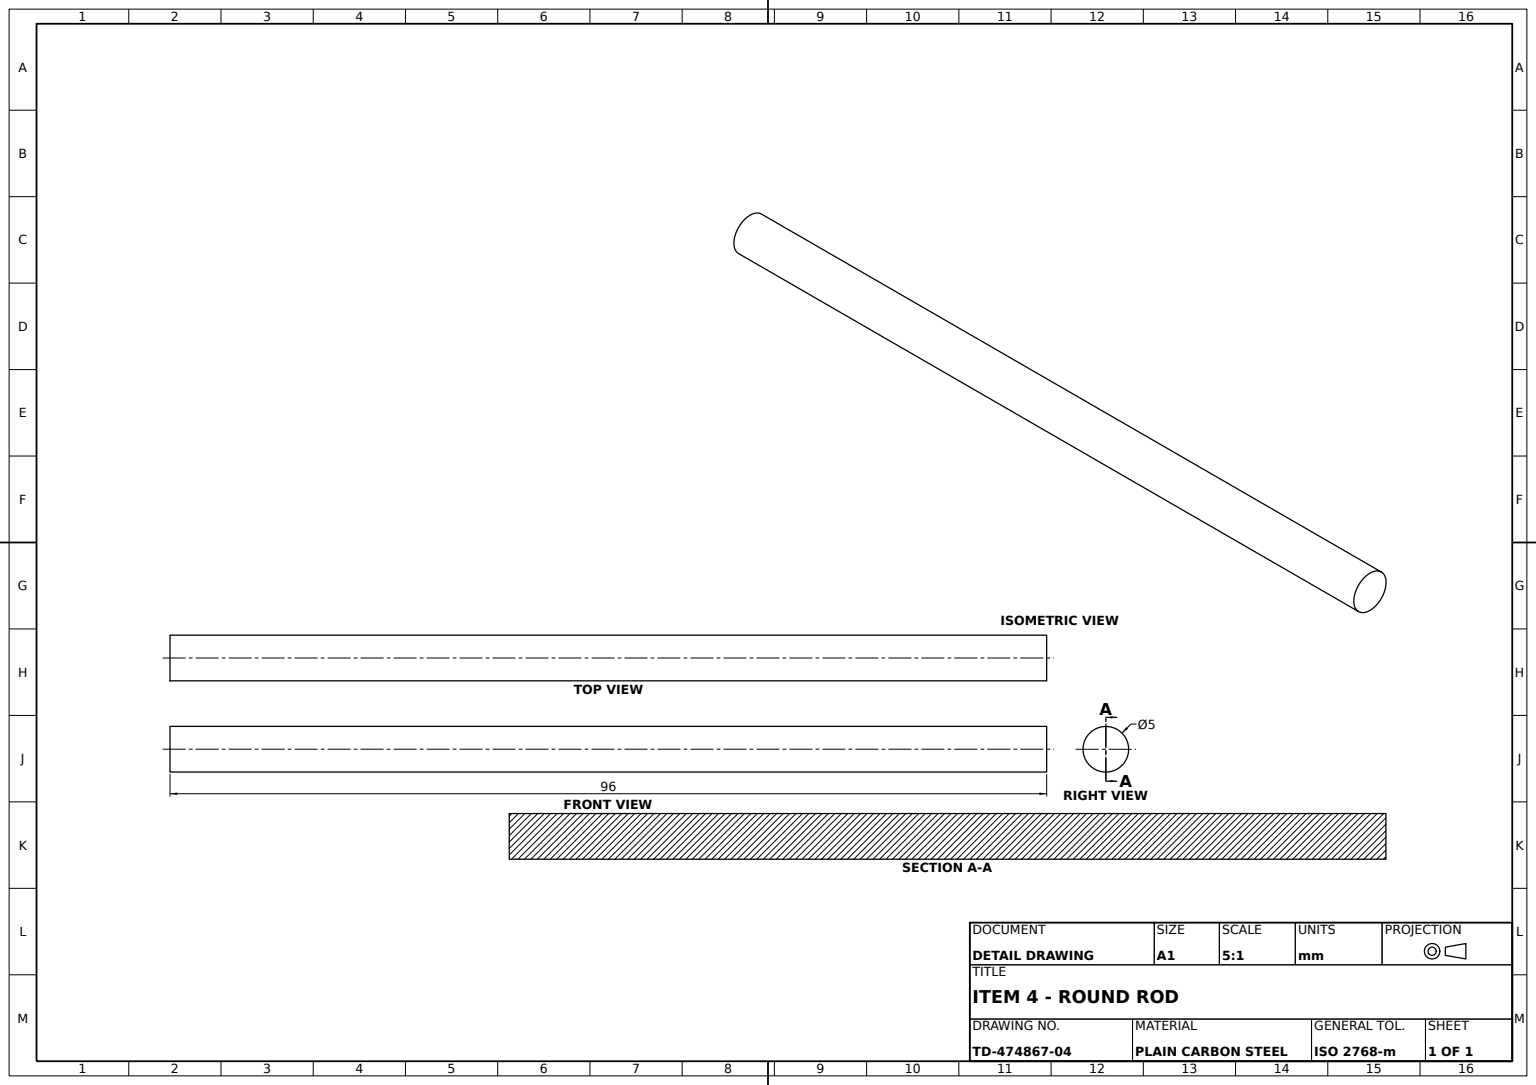
ISO-10303-21;
HEADER;
FILE_DESCRIPTION((''),'2;1');
FILE_NAME('','',(''),(''),'','','');
FILE_SCHEMA(('AUTOMOTIVE_DESIGN'));
ENDSEC;
DATA;
#1=APPLICATION_CONTEXT('');
#2=PRODUCT_CONTEXT('',#1,'mechanical');
#3=PRODUCT('','','',(#2));
#4=PRODUCT_DEFINITION_FORMATION('','',#3);
#5=PRODUCT_DEFINITION_CONTEXT('',#1,'design');
#6=PRODUCT_DEFINITION('','',#4,#5);
#7=PRODUCT_DEFINITION_SHAPE('','',#6);
#8=(LENGTH_UNIT()NAMED_UNIT(*)SI_UNIT(.MILLI.,.METRE.));
#9=(NAMED_UNIT(*)PLANE_ANGLE_UNIT()SI_UNIT($,.RADIAN.));
#10=(NAMED_UNIT(*)SI_UNIT($,.STERADIAN.)SOLID_ANGLE_UNIT());
#11=UNCERTAINTY_MEASURE_WITH_UNIT(LENGTH_MEASURE(1.E-05),#8,'distance_accuracy_value','');
#12=(GEOMETRIC_REPRESENTATION_CONTEXT(3)GLOBAL_UNCERTAINTY_ASSIGNED_CONTEXT((#11))GLOBAL_UNIT_ASSIGNED_CONTEXT((#8,#9,#10))REPRESENTATION_CONTEXT('',''));
#13=CARTESIAN_POINT('',(-2.5,0.,-48.));
#14=VERTEX_POINT('',#13);
#15=CARTESIAN_POINT('',(2.5,0.,-48.));
#16=VERTEX_POINT('',#15);
#17=CARTESIAN_POINT('',(0.,0.,-48.));
#18=DIRECTION('',(0.,0.,1.));
#19=DIRECTION('',(1.,0.,0.));
#20=AXIS2_PLACEMENT_3D('',#17,#18,#19);
#21=CIRCLE('',#20,2.5);
#22=EDGE_CURVE('',#14,#16,#21,.T.);
#23=ORIENTED_EDGE('',*,*,#22,.F.);
#24=EDGE_CURVE('',#16,#14,#21,.T.);
#25=ORIENTED_EDGE('',*,*,#24,.F.);
#26=EDGE_LOOP('',(#23,#25));
#27=FACE_OUTER_BOUND('',#26,.T.);
#28=PLANE('',#20);
#29=ADVANCED_FACE('',(#27),#28,.F.);
#30=CARTESIAN_POINT('',(-2.5,0.,48.));
#31=VERTEX_POINT('',#30);
#32=DIRECTION('',(0.,0.,-1.));
#33=VECTOR('',#32,1000.);
#34=LINE('',#30,#33);
#35=EDGE_CURVE('',#31,#14,#34,.T.);
#36=ORIENTED_EDGE('',*,*,#35,.F.);
#37=CARTESIAN_POINT('',(2.5,0.,48.));
#38=VERTEX_POINT('',#37);
#39=CARTESIAN_POINT('',(0.,0.,48.));
#40=AXIS2_PLACEMENT_3D('',#39,#18,#19);
#41=CIRCLE('',#40,2.5);
#42=EDGE_CURVE('',#38,#31,#41,.T.);
#43=ORIENTED_EDGE('',*,*,#42,.F.);
#44=LINE('',#37,#33);
#45=EDGE_CURVE('',#38,#16,#44,.T.);
#46=ORIENTED_EDGE('',*,*,#45,.T.);
#47=ORIENTED_EDGE('',*,*,#24,.T.);
#48=EDGE_LOOP('',(#36,#43,#46,#47));
#49=FACE_OUTER_BOUND('',#48,.T.);
#50=DIRECTION('',(-1.,0.,0.));
#51=AXIS2_PLACEMENT_3D('',#39,#32,#50);
#52=CYLINDRICAL_SURFACE('',#51,2.5);
#53=ADVANCED_FACE('',(#49),#52,.T.);
#54=ORIENTED_EDGE('',*,*,#35,.T.);
#55=ORIENTED_EDGE('',*,*,#22,.T.);
#56=ORIENTED_EDGE('',*,*,#45,.F.);
#57=EDGE_CURVE('',#31,#38,#41,.T.);
#58=ORIENTED_EDGE('',*,*,#57,.F.);
#59=EDGE_LOOP('',(#54,#55,#56,#58));
#60=FACE_OUTER_BOUND('',#59,.T.);
#61=ADVANCED_FACE('',(#60),#52,.T.);
#62=ORIENTED_EDGE('',*,*,#42,.T.);
#63=ORIENTED_EDGE('',*,*,#57,.T.);
#64=EDGE_LOOP('',(#62,#63));
#65=FACE_OUTER_BOUND('',#64,.T.);
#66=PLANE('',#40);
#67=ADVANCED_FACE('',(#65),#66,.T.);
#68=CLOSED_SHELL('',(#29,#53,#61,#67));
#69=MANIFOLD_SOLID_BREP('',#68);
#70=ADVANCED_BREP_SHAPE_REPRESENTATION('',(#69),#12);
#71=SHAPE_DEFINITION_REPRESENTATION(#7,#70);
ENDSEC;
END-ISO-10303-21;
